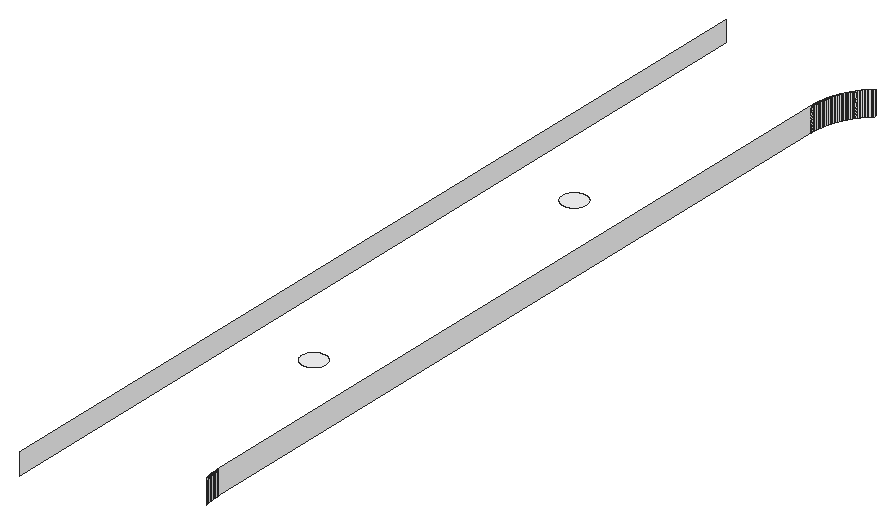
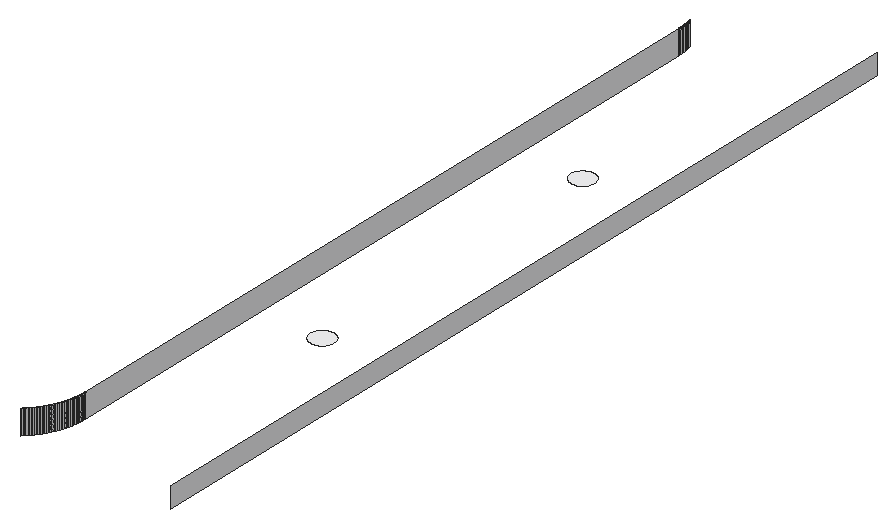
# SketchUp Ruby script. Lengths in inches.
U = 1.inch
M = Sketchup.active_model
def pt(a) = Geom::Point3d.new(a.map { |v| v * U })
def face(e, loops, mat)
  f = e.add_face(loops[0].map { |a| pt(a) })
  loops[1..].each { |l| e.add_face(l.map { |a| pt(a) }).erase! }
  f.material = f.back_material = mat if mat
  f
end
# faces: each face lists its corners as indices into pts; further lists are holes
def faces(e, pts, list, mat = nil) = list.each { |f| face(e, (f[0].is_a?(Array) ? f : [f]).map { |l| l.map { |i| pts[i] } }, mat) }
# xy, xz, yz: faces in a plane at the given z, y or x. An outline is a flat list of corners, or four numbers for a rectangle; further outlines are holes
def ring(l) = l.size == 4 ? [[l[0], l[1]], [l[2], l[1]], [l[2], l[3]], [l[0], l[3]]] : l.each_slice(2).to_a
def flat(e, list, mat, &to3) = list.each { |f| face(e, (f[0].is_a?(Array) ? f : [f]).map { |l| ring(l).map { |u, v| to3.(u, v) } }, mat) }
def xy(e, z, list, mat = nil) = flat(e, list, mat) { |x, y| [x, y, z] }
def xz(e, y, list, mat = nil) = flat(e, list, mat) { |x, z| [x, y, z] }
def yz(e, x, list, mat = nil) = flat(e, list, mat) { |y, z| [x, y, z] }
def lines(e, pts, list) = list.each { |a, b| e.add_line(pt(pts[a]), pt(pts[b])) }
# prism: a flat outline (further loops are holes) pulled along v
def prism(e, loops, v, mat = nil)
  f = face(e, loops, mat); d = Geom::Vector3d.new(v.map { |x| x * U })
  f.pushpull(f.normal.samedirection?(d) ? d.length : -d.length)
end
def box(e, o, s, mat = nil) = prism(e, [[o, [o[0] + s[0], o[1], o[2]], [o[0] + s[0], o[1] + s[1], o[2]], [o[0], o[1] + s[1], o[2]]]], [0, 0, s[2]], mat)
def at(x, y, z, deg = 0) = Geom::Transformation.translation(pt([x, y, z])) * Geom::Transformation.rotation(ORIGIN, Z_AXIS, deg.degrees)
def axes(o, x, y, z) = Geom::Transformation.new([*x, 0, *y, 0, *z, 0, *pt(o).to_a, 1])
def part(name) = M.definitions.add(name)
# library, detail: a bought-in or finely detailed component or shape, given as its bounding box
def library(name, o, s) = part(name).tap { |d| box(d.entities, o, s) }
def detail(e, o, s) = box(e.add_group.entities, o, s)
def put(e, d, t, mat = nil) = e.add_instance(d, t).tap { |i| i.material = mat if mat }
def group(e, t, mat = nil) = e.add_group.tap { |g| g.transformation = t; g.material = mat if mat }.entities
root = M.entities
M.materials.add("[Quartz Light Grey]").color = [251, 251, 252]
xy(root,112.81,[[33.02,111.35,32.9,111.36,32.77,111.37,32.65,111.39,32.52,111.41,32.28,111.49,32.06,111.59,31.95,111.65,31.84,111.72,31.74,111.8,31.65,111.88,31.56,111.97,31.47,112.0625,31.39,112.16,31.32,112.26,31.2,112.48,31.1,112.72,31.04,112.96,31.02,113.08,31.01,113.21,31,113.33,31,113.46,31.01,113.58,31.03,113.71,31.09,113.95,31.13,114.07,31.18,114.1875,31.24,114.3,31.3,114.41,31.37,114.51,31.53,114.71,31.62,114.8,31.71,114.88,31.81,114.96,31.91,115.03,32.02,115.1,32.13,115.15,32.24,115.21,32.48,115.29,32.6,115.31,32.73,115.34,32.85,115.35,33.1,115.35,33.23,115.34,33.35,115.32,33.48,115.3,33.72,115.22,33.94,115.12,34.16,114.98,34.26,114.91,34.35,114.83,34.53,114.65,34.61,114.55,34.68,114.44,34.74,114.34,34.8,114.23,34.9,113.99,34.96,113.75,34.98,113.625,35,113.375,35,113.25,34.99,113.125,34.97,113,34.91,112.76,34.87,112.64,34.82,112.52,34.7,112.3,34.63,112.2,34.47,112,34.38,111.91,34.29,111.83,34.19,111.75,34.09,111.68,33.98,111.61,33.87,111.55,33.76,111.5,33.52,111.42,33.4,111.39,33.27,111.37,33.15,111.36],[32.9,166.71,32.77,166.72,32.65,166.74,32.52,166.77,32.4,166.8,32.28,166.84,32.17,166.89,31.95,167.01,31.84,167.08,31.74,167.15,31.65,167.24,31.56,167.32,31.47,167.42,31.39,167.52,31.32,167.62,31.2,167.84,31.15,167.95,31.1,168.07,31.07,168.19,31.04,168.3125,31.02,168.4375,31,168.6875,31,168.8125,31.01,168.9375,31.03,169.0625,31.06,169.19,31.09,169.31,31.13,169.42,31.18,169.54,31.3,169.76,31.37,169.87,31.45,169.97,31.53,170.0625,31.62,170.15,31.71,170.24,31.81,170.3125,31.91,170.39,32.13,170.51,32.24,170.56,32.48,170.64,32.6,170.67,32.73,170.69,32.85,170.7,32.98,170.71,33.1,170.71,33.23,170.7,33.35,170.68,33.48,170.65,33.6,170.62,33.72,170.58,33.83,170.53,34.05,170.41,34.16,170.34,34.26,170.26,34.35,170.18,34.53,170,34.61,169.9,34.68,169.8,34.8,169.58,34.85,169.46,34.9,169.35,34.93,169.23,34.96,169.1,34.98,168.98,34.99,168.86,35,168.73,35,168.6,34.99,168.48,34.97,168.35,34.91,168.11,34.87,167.99,34.82,167.875,34.76,167.76,34.7,167.66,34.63,167.55,34.55,167.45,34.47,167.36,34.29,167.18,34.19,167.1,34.09,167.03,33.87,166.91,33.76,166.86,33.64,166.8125,33.52,166.78,33.4,166.75,33.27,166.73,33.15,166.71]],"[Quartz Light Grey]")
yz(root,21,[[66,111.81,216,115.32]],"[Quartz Light Grey]")
yz(root,45,[[77.75,111.81,77.91,115.91],[77.91,111.81,78.0625,115.91],[78.0625,111.81,204,115.91],[204,111.81,204.16,115.91],[204.16,111.81,204.3125,115.91]],"[Quartz Light Grey]")
yz(root,45.01,[[77.43,111.81,77.59,115.91]],"[Quartz Light Grey]")
p = [[45.32,75.25,111.81],[45.28,75.4,111.81],[45.28,75.4,115.91],[45.32,75.25,115.91],[45.25,75.56,111.81],[45.25,75.56,115.91],
  [45.22,75.71,111.81],[45.22,75.71,115.91],[45.19,75.87,111.81],[45.19,75.87,115.91],[45.16,76.02,111.81],[45.16,76.02,115.91],
  [45.14,76.18,111.81],[45.14,76.18,115.91],[45.12,76.33,111.81],[45.12,76.33,115.91],[45.1,76.49,111.81],[45.1,76.49,115.91],
  [45.08,76.65,111.81],[45.08,76.65,115.91],[45.06,76.8,111.81],[45.06,76.8,115.91],[45.04,76.96,111.81],[45.04,76.96,115.91],
  [45.03,77.12,111.81],[45.03,77.12,115.91],[45.02,77.28,111.81],[45.02,77.28,115.91],[45.01,77.43,111.81],[45.01,77.43,115.91],
  [45.01,77.59,111.81],[45,77.75,111.81],[45,77.75,115.91],[45.01,77.59,115.91],[45,204.3125,111.81],[45.01,204.47,111.81],
  [45.01,204.47,115.91],[45,204.3125,115.91],[45.02,204.63,111.81],[45.02,204.63,115.91],[45.03,204.78,111.81],[45.03,204.78,115.91],
  [45.04,204.94,111.81],[45.04,204.94,115.91],[45.05,205.1,111.81],[45.05,205.1,115.91],[45.07,205.25,111.81],[45.07,205.25,115.91],
  [45.08,205.41,111.81],[45.08,205.41,115.91],[45.1,205.57,111.81],[45.1,205.57,115.91],[45.125,205.72,111.81],[45.125,205.72,115.91],
  [45.15,205.88,111.81],[45.15,205.88,115.91],[45.17,206.03,111.81],[45.17,206.03,115.91],[45.2,206.1875,111.81],[45.2,206.1875,115.91],
  [45.23,206.34,111.81],[45.23,206.34,115.91],[45.26,206.49,111.81],[45.26,206.49,115.91],[45.3,206.65,111.81],[45.3,206.65,115.91],
  [45.33,206.8,111.81],[45.33,206.8,115.91],[45.37,206.95,111.81],[45.37,206.95,115.91],[45.41,207.11,111.81],[45.41,207.11,115.91],
  [45.45,207.26,111.81],[45.45,207.26,115.91],[45.49,207.41,111.81],[45.49,207.41,115.91],[45.54,207.56,111.81],[45.54,207.56,115.91],
  [45.59,207.71,111.81],[45.59,207.71,115.91],[45.64,207.86,111.81],[45.64,207.86,115.91],[45.6875,208.01,111.81],[45.6875,208.01,115.91],
  [45.74,208.15,111.81],[45.74,208.15,115.91],[45.8,208.3,111.81],[45.8,208.3,115.91],[45.85,208.45,111.81],[45.85,208.45,115.91],
  [45.91,208.59,111.81],[45.91,208.59,115.91],[45.97,208.74,111.81],[45.97,208.74,115.91],[46.04,208.88,111.81],[46.04,208.88,115.91],
  [46.1,209.02,111.81],[46.1,209.02,115.91],[46.17,209.17,111.81],[46.17,209.17,115.91],[46.24,209.31,111.81],[46.24,209.31,115.91],
  [46.31,209.45,111.81],[46.31,209.45,115.91],[46.38,209.59,111.81],[46.38,209.59,115.91],[46.45,209.73,111.81],[46.45,209.73,115.91],
  [46.53,209.86,111.81],[46.53,209.86,115.91],[46.61,210,111.81],[46.61,210,115.91],[46.6875,210.14,111.81],[46.6875,210.14,115.91],
  [46.77,210.27,111.81],[46.77,210.27,115.91],[46.85,210.4,111.81],[46.85,210.4,115.91],[46.9375,210.54,111.81],[46.9375,210.54,115.91],
  [47.02,210.67,111.81],[47.02,210.67,115.91],[47.11,210.8,111.81],[47.11,210.8,115.91],[47.2,210.93,111.81],[47.2,210.93,115.91],
  [47.29,211.05,111.81],[47.29,211.05,115.91],[47.38,211.18,111.81],[47.38,211.18,115.91],[47.48,211.31,111.81],[47.48,211.31,115.91],
  [47.58,211.43,111.81],[47.58,211.43,115.91],[47.67,211.55,111.81],[47.67,211.55,115.91],[47.77,211.67,111.81],[47.77,211.67,115.91],
  [47.875,211.79,111.81],[47.875,211.79,115.91],[47.98,211.91,111.81],[47.98,211.91,115.91],[48.08,212.03,111.81],[48.08,212.03,115.91],
  [48.1875,212.15,111.81],[48.1875,212.15,115.91],[48.3,212.26,111.81],[48.3,212.26,115.91],[48.4,212.375,111.81],[48.4,212.375,115.91],
  [48.51,212.49,111.81],[48.51,212.49,115.91],[48.625,212.6,111.81],[48.625,212.6,115.91],[48.74,212.7,111.81],[48.74,212.7,115.91],
  [48.85,212.8125,111.81],[48.85,212.8125,115.91],[48.97,212.92,111.81],[48.97,212.92,115.91]]
faces(root,p,[[0,1,2,3],[1,4,5,2],[4,6,7,5],[6,8,9,7],[8,10,11,9],[10,12,13,11],[12,14,15,13],[14,16,17,15],
  [16,18,19,17],[18,20,21,19],[20,22,23,21],[22,24,25,23],[24,26,27,25],[26,28,29,27],[30,31,32,33],[34,35,36,37],
  [35,38,39,36],[38,40,41,39],[40,42,43,41],[42,44,45,43],[44,46,47,45],[46,48,49,47],[48,50,51,49],[50,52,53,51],
  [52,54,55,53],[54,56,57,55],[56,58,59,57],[58,60,61,59],[60,62,63,61],[62,64,65,63],[64,66,67,65],[66,68,69,67],
  [68,70,71,69],[70,72,73,71],[72,74,75,73],[74,76,77,75],[76,78,79,77],[78,80,81,79],[80,82,83,81],[82,84,85,83],
  [84,86,87,85],[86,88,89,87],[88,90,91,89],[90,92,93,91],[92,94,95,93],[94,96,97,95],[96,98,99,97],[98,100,101,99],
  [100,102,103,101],[102,104,105,103],[104,106,107,105],[106,108,109,107],[108,110,111,109],[110,112,113,111],[112,114,115,113],[114,116,117,115],
  [116,118,119,117],[118,120,121,119],[120,122,123,121],[122,124,125,123],[124,126,127,125],[126,128,129,127],[128,130,131,129],[130,132,133,131],
  [132,134,135,133],[134,136,137,135],[136,138,139,137],[138,140,141,139],[140,142,143,141],[142,144,145,143],[144,146,147,145],[146,148,149,147],
  [148,150,151,149],[150,152,153,151],[152,154,155,153],[154,156,157,155],[156,158,159,157]],"[Quartz Light Grey]")
